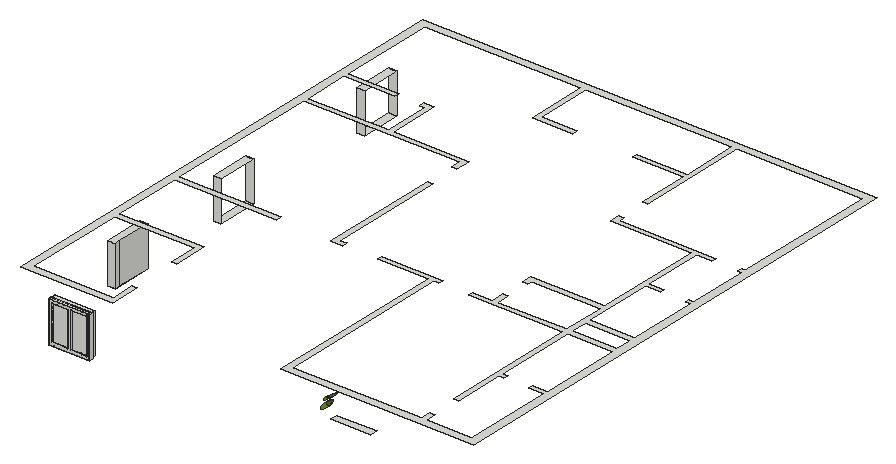
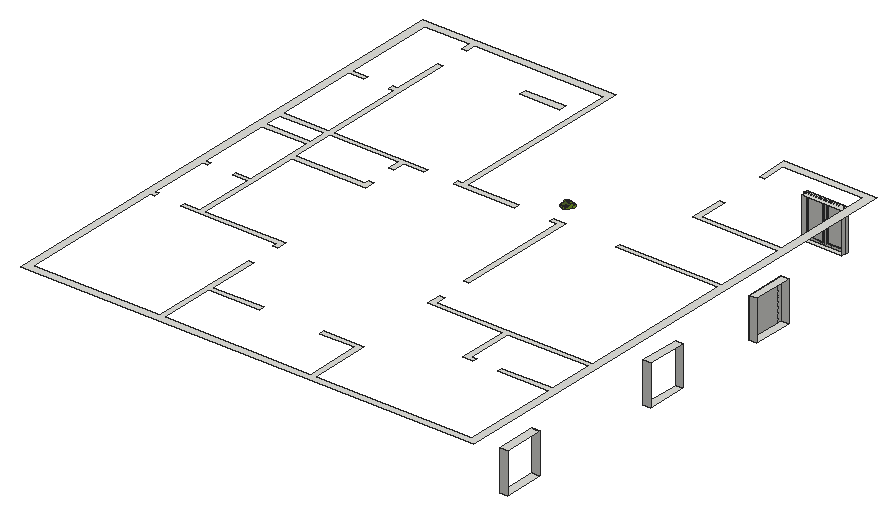
# SketchUp Ruby script. Lengths in inches.
U = 1.inch
M = Sketchup.active_model
def pt(a) = Geom::Point3d.new(a.map { |v| v * U })
def face(e, loops, mat)
  f = e.add_face(loops[0].map { |a| pt(a) })
  loops[1..].each { |l| e.add_face(l.map { |a| pt(a) }).erase! }
  f.material = f.back_material = mat if mat
  f
end
# faces: each face lists its corners as indices into pts; further lists are holes
def faces(e, pts, list, mat = nil) = list.each { |f| face(e, (f[0].is_a?(Array) ? f : [f]).map { |l| l.map { |i| pts[i] } }, mat) }
# xy, xz, yz: faces in a plane at the given z, y or x. An outline is a flat list of corners, or four numbers for a rectangle; further outlines are holes
def ring(l) = l.size == 4 ? [[l[0], l[1]], [l[2], l[1]], [l[2], l[3]], [l[0], l[3]]] : l.each_slice(2).to_a
def flat(e, list, mat, &to3) = list.each { |f| face(e, (f[0].is_a?(Array) ? f : [f]).map { |l| ring(l).map { |u, v| to3.(u, v) } }, mat) }
def xy(e, z, list, mat = nil) = flat(e, list, mat) { |x, y| [x, y, z] }
def xz(e, y, list, mat = nil) = flat(e, list, mat) { |x, z| [x, y, z] }
def yz(e, x, list, mat = nil) = flat(e, list, mat) { |y, z| [x, y, z] }
def lines(e, pts, list) = list.each { |a, b| e.add_line(pt(pts[a]), pt(pts[b])) }
# prism: a flat outline (further loops are holes) pulled along v
def prism(e, loops, v, mat = nil)
  f = face(e, loops, mat); d = Geom::Vector3d.new(v.map { |x| x * U })
  f.pushpull(f.normal.samedirection?(d) ? d.length : -d.length)
end
def box(e, o, s, mat = nil) = prism(e, [[o, [o[0] + s[0], o[1], o[2]], [o[0] + s[0], o[1] + s[1], o[2]], [o[0], o[1] + s[1], o[2]]]], [0, 0, s[2]], mat)
def at(x, y, z, deg = 0) = Geom::Transformation.translation(pt([x, y, z])) * Geom::Transformation.rotation(ORIGIN, Z_AXIS, deg.degrees)
def axes(o, x, y, z) = Geom::Transformation.new([*x, 0, *y, 0, *z, 0, *pt(o).to_a, 1])
def part(name) = M.definitions.add(name)
# library, detail: a bought-in or finely detailed component or shape, given as its bounding box
def library(name, o, s) = part(name).tap { |d| box(d.entities, o, s) }
def detail(e, o, s) = box(e.add_group.entities, o, s)
def put(e, d, t, mat = nil) = e.add_instance(d, t).tap { |i| i.material = mat if mat }
def group(e, t, mat = nil) = e.add_group.tap { |g| g.transformation = t; g.material = mat if mat }.entities
root = M.entities
M.materials.add("[0059_DarkOliveGreen]").color = [85, 107, 47]
M.materials.add("[0061_OliveDrab]").color = [107, 142, 35]
c1 = part("Window")
xy(c1.entities,31.72,[[-0.78,88.6,2.72,128.1]])
xy(c1.entities,34.95,[[-0.78,91.53,0.84,106.59],[0.84,91.53,1.05,97.58],[1.05,91.53,1.42,106.59],[1.42,91.53,2.72,106.59],[0.84,97.58,1.05,98.18],
  [0.84,98.18,1.05,106.59]])
xy(c1.entities,35.27,[[-0.78,110.09,0.97,125.14],[1.05,110.09,2.72,125.14]])
xy(c1.entities,58.35,[[2.72,108.74,3.8,109.74]])
xy(c1.entities,77.8125,[[-0.78,110.09,2.72,125.14],[0.97,110.09,1.05,125.14]])
xy(c1.entities,77.93,[[-0.78,91.53,0.84,106.59],[1.05,91.53,1.42,106.59],[1.42,91.53,2.72,106.59]])
xy(c1.entities,80.72,[[-0.78,88.6,2.72,128.1]])
xz(c1.entities,88.6,[[-0.78,31.72,2.72,80.72]])
xz(c1.entities,91.53,[[-0.78,34.95,0.84,77.93],[1.05,34.95,1.42,77.93],[1.42,34.95,2.72,77.93]])
xz(c1.entities,106.59,[[-0.78,34.95,0.84,77.93],[0.84,34.95,1.05,77.93],[0.84,34.95,2.72,77.93]])
xz(c1.entities,108.74,[[3.8,54.35,4.22,54.6,4.22,59.47,2.72,59.97,2.72,58.35,3.8,58.35]])
xz(c1.entities,109.74,[[3.8,54.35,3.8,58.35,2.72,58.35,2.72,59.97,4.22,59.47,4.22,54.6]])
xz(c1.entities,110.09,[[-0.78,35.27,0.97,77.8125],[1.05,35.27,2.72,77.8125]])
xz(c1.entities,125.14,[[-0.78,35.27,0.97,77.8125],[0.97,35.27,1.05,80.72],[1.05,35.27,2.72,77.8125]])
xz(c1.entities,128.1,[[-0.78,31.72,2.72,80.72]])
yz(c1.entities,-0.78,[[[88.6,31.72,128.1,80.72],[91.53,34.95,106.59,77.93],[110.09,35.27,125.14,77.8125]]])
yz(c1.entities,0.84,[[91.53,34.95,106.59,77.93]])
yz(c1.entities,0.97,[[110.09,35.27,125.14,77.8125]])
yz(c1.entities,1.05,[[91.53,34.95,106.59,77.93],[110.09,35.27,125.14,77.8125]])
yz(c1.entities,1.42,[[91.53,34.95,106.59,77.93]])
yz(c1.entities,2.72,[[[88.6,31.72,108.35,80.72],[91.53,34.95,106.59,77.93]],[[108.35,31.72,128.1,80.72],[110.09,35.27,125.14,77.8125],[108.74,58.35,109.74,59.97]]])
yz(c1.entities,3.8,[[108.74,54.35,109.74,58.35]])
yz(c1.entities,4.22,[[108.74,54.6,109.74,59.47]])
p = [[4.22,108.74,54.6],[3.8,108.74,54.35],[3.8,109.74,54.35],[4.22,109.74,54.6],[2.72,109.74,59.97],[2.72,108.74,59.97],
  [4.22,108.74,59.47],[4.22,109.74,59.47],[-0.78,86.4,89.94],[-0.78,86.44,89.94],[15.22,130.69,89.94],[15.22,130.65,89.94],
  [-0.78,86.44,28.19],[-0.78,86.4,28.19],[7.72,130.69,89.94],[7.72,130.65,89.94]]
faces(c1.entities,p,[[0,1,2,3],[4,5,6,7]])
lines(c1.entities,p,[[8,9],[10,11],[12,13],[14,15]])
xy(root,30.79,[[0,130.58,9,178.58],[0,288.02,9,336.02],[0,501.46,9,549.46]])
xy(root,38.11,[[33.63,0,81.63,9]])
xy(root,75.37,[[370.05,0,418.05,9]])
xy(root,78.79,[[0,130.58,9,178.58],[0,288.02,9,336.02],[0,501.46,9,549.46]])
xy(root,86.11,[[33.63,0,81.63,9]])
xy(root,108,[[[0,0,110,0,110,36.625,104,36.625,104,9,9,9,9,130,104,130,104,95.625,110,95.625,110,136,9,136,9,219,130,219,130,225,9,225,9,411,195,411,195,399,201,399,201,417,111,417,111,477,99,477,99,471,105,471,105,417,9,417,9,471,69,471,69,477,9,477,9,591,195,591,195,519,243.14,519,243.14,525,201,525,201,591,375,591,375,525,315.14,525,315.14,519,375,519,375,459,381,459,381,591,531,591,531,417,526.66,417,526.66,411,531,411,531,340,525,340,525,335,531,335,531,252,477,252,477,335,495,335,495,340,477,340,477,411,495.74,411,495.74,417,381,417,381,423,375,423,375,411,471,411,471,282,383,282,383,270,389,270,389,276,471,276,471,225,389,225,389,240,383,240,383,225,359,225,359,219,471,219,471,57,477,57,477,116,483,116,483,122,477,122,477,219,531,219,531,122,513,122,513,116,531,116,531,9,477,9,477,21,471,21,471,9,317,9,317,219,323,219,323,225,250.53,225,250.53,219,311,219,311,0,540,0,540,600,0,600],[477,225,531,246]],[195,219,208.87,219,208.87,225,201,225,201,363,195,363]])
xz(root,130.58,[[0,30.79,9,78.79]])
xz(root,178.58,[[0,30.79,9,78.79]])
xz(root,288.02,[[0,30.79,9,78.79]])
xz(root,336.02,[[0,30.79,9,78.79]])
xz(root,501.46,[[0,30.79,9,78.79]])
xz(root,549.46,[[0,30.79,9,78.79]])
yz(root,9,[[130.58,30.79,136,78.79],[136,30.79,178.58,78.79]])
yz(root,33.63,[[0,38.11,9,86.11]])
yz(root,81.63,[[0,38.11,9,86.11]])
p = [[303.91,81.51,31.81],[304.14,80.48,31.67],[304.01,79.54,31.42],[303.76,79.01,31.21],[303.29,78.55,30.94],[303.13,78.34,30.84],
  [303.1,79.46,31.08],[302.88,80.62,31.25],[302.55,81.73,31.37],[302.14,82.53,31.4],[302.01,82.68,31.38],[301.96,82.62,31.35],
  [302.02,82.34,31.3125],[302.4375,81.03,31.18],[302.71,79.875,31.03],[302.94,78.63,30.84],[303.01,77.97,30.72],[302.91,77.39,30.56],
  [302.67,77.08,30.41],[302.28,76.75,30.2],[301.93,76.47,30.01],[301.74,76.33,29.91],[301.4375,75.8125,29.69],[301.09,75.45,29.49],
  [300.73,75.23,29.31],[300.54,75.08,29.21],[300.5625,75.71,29.36],[300.6,76.66,29.57],[300.24,74.96,29.08],[300.13,74.76,29],
  [299.8,74.7,28.87],[299.47,74.65,28.73],[298.7,75.08,28.56],[297.62,75.29,28.21],[297.18,76.34,28.29],[296.74,77.08,28.29],
  [296.46,77.49,28.28],[297.01,78.56,28.7],[297.43,79.14,28.98],[298.05,79.55,29.29],[298.48,79.8,29.5],[298.6875,80.09,29.64],
  [298.86,80.33,29.75],[298.86,80.48,29.78],[298.74,80.54,29.75],[298.4,80.41,29.6],[298.12,80.21,29.46],[297.52,79.55,29.1],
  [297.02,78.96,28.8],[296.71,78.63,28.61],[296.5,78.25,28.46],[296.35,77.84,28.3125],[296.125,78.48,28.37],[296.02,79.02,28.45],
  [295.96,79.5,28.53],[295.9375,79.89,28.61],[295.88,80.34,28.6875],[296.37,81.17,29.04],[296.83,81.62,29.3],[297.24,81.82,29.49],
  [298,82.06,29.8125],[298.57,82.12,30.03],[299.0625,82.22,30.23],[299.42,82.36,30.39],[299.6,82.6,30.5],[299.61,82.92,30.58],
  [299.33,83.05,30.51],[298.96,83.14,30.39],[298.31,82.98,30.125],[297.6,82.57,29.78],[296.82,81.9375,29.37],[295.94,80.96,28.84],
  [295.84,82.59,29.16],[295.83,83.55,29.36],[295.97,83.97,29.5],[296.29,84.41,29.71],[296.68,84.67,29.91],[297.22,84.77,30.12],
  [297.67,84.84,30.3],[298.34,84.92,30.56],[298.83,84.87,30.72],[299.22,84.82,30.85],[299.41,84.76,30.9],[299.52,84.91,30.97],
  [299.4,85.13,30.98],[299.12,85.42,30.94],[298.67,85.56,30.8125],[297.76,85.4375,30.46],[297.22,85.26,30.23],[296.75,85.02,30.01],
  [296.53,84.79,29.88],[296.09,84.42,29.64],[296.07,84.68,29.7],[296.18,85.62,29.9375],[296.3,86.45,30.16],[296.74,87.4,30.52],
  [297.2,87.58,30.72],[297.94,87.44,30.96],[298.59,87.05,31.11],[299.19,86.76,31.26],[299.45,86.61,31.32],[299.6,86.64,31.38],
  [299.58,86.81,31.41],[299.28,87.16,31.38],[298.55,87.65,31.22],[297.96,87.8,31.04],[297.01,87.79,30.71],[297.49,88.92,31.12],
  [297.97,89.5,31.42],[298.37,89.6,31.58],[298.58,89.41,31.61],[299.21,88.79,31.7],[299.67,88.22,31.75],[300.03,87.86,31.8],
  [300.18,87.82,31.84],[300.22,87.97,31.89],[300.15,88.13,31.9],[299.5625,88.88,31.85],[299.09,89.3125,31.78],[298.68,89.59,31.6875],
  [298.36,89.78,31.62],[298.75,90.2,31.85],[299.11,90.32,32],[299.58,90.14,32.13],[300.02,89.78,32.21],[300.47,89.53,32.32],
  [300.7,89.07,32.3],[301.09,88.52,32.32],[301.42,87.875,32.3],[301.58,87.02,32.17],[301.53,86.13,31.96],[301.42,85.61,31.81],
  [301.65,85.42,31.85],[301.84,85.85,32.01],[302.16,86.29,32.22],[302.57,86.26,32.36],[303.18,85.93,32.5],[303.73,85.6,32.63],
  [304.125,85.47,32.74],[304.36,83.6,32.42],[304.35,82.48,32.17],[304.15,81.83,31.96],[302.35,78.69,30.64],[302.07,81.12,31.07],
  [301.58,82.73,31.24],[301.05,84.09,31.35],[301.19,84.49,31.48],[301.73,83.94,31.56],[302.45,83.22,31.66],[303.17,81.58,31.56],
  [302.67,83.06,31.7],[302.11,84.15,31.74],[301.47,84.58,31.6],[301.37,84.78,31.61],[301.58,85.07,31.75],[302.58,84.5,31.98],
  [303.72,84.24,32.33],[301.46,85.37,31.77],[301.27,86.02,31.84],[300.98,87.4375,32.04],[300.59,88.32,32.1],[300.25,88.84,32.09],
  [300.78,87.35,31.95],[301.08,86.13,31.8],[301.18,85.44,31.68],[300.75,86.54,31.77],[299.91,87.57,31.6875],[299.23,88.12,31.57],
  [298.53,88.54,31.41],[298.19,88.67,31.3125],[299.26,87.8125,31.51],[299.9,87.21,31.61],[300.61,86.39,31.68],[300.97,85.68,31.66],
  [301.12,85.28,31.63],[301.09,85.03,31.5625],[300.97,84.97,31.51],[300.66,85.21,31.45],[300.34,85.6,31.42],[299.97,85.85,31.34],
  [298.9,86.35,31.07],[298.22,86.5,30.86],[297.58,86.36,30.6],[297.06,86.27,30.39],[296.86,86,30.26],[297.86,86.19,30.66],
  [298.43,86.13,30.85],[299.33,85.85,31.11],[300.12,85.39,31.29],[300.98,84.75,31.46],[300.53,83.74,31.08],[299.86,83.98,30.9],
  [299.23,84.18,30.72],[297.93,83.99,30.21],[297.28,83.64,29.9],[296.85,83.33,29.68],[296.65,83.05,29.55],[297.26,83.38,29.84],
  [298.27,83.68,30.26],[299.56,83.77,30.74],[300.33,83.47,30.95],[299.64,81.54,30.29],[299.12,81.68,30.13],[298.48,81.48,29.86],
  [297.875,81.06,29.55],[297.41,80.6,29.29],[296.91,79.91,28.96],[297.95,80.89,29.54],[298.56,81.28,29.85],[299.12,81.41,30.08],
  [299.63,81.3125,30.24],[299.19,79.81,29.75],[298.63,79.54,29.5],[298.13,79.07,29.22],[297.72,78.51,28.95],[297.54,77.96,28.76],
  [298.23,78.9,29.21],[298.74,79.27,29.48],[299.16,79.49,29.67],[298.73,78.33,29.27],[298.51,77.7,29.05],[298.1875,76.91,28.77],
  [298.25,77.01,28.81],[298.86,78.18,29.28],[299.35,79.38,29.72],[299.73,80.8,30.16],[299.98,77.43,29.52],[299.97,81.28,30.35],
  [300.41,82.42,30.76],[300.8125,80.77,30.54],[301.22,78.1,30.11],[301.07,80.07,30.48],[300.77,81.88,30.77],[300.53,82.84,30.89],
  [300.96,83.8,31.25],[301.66,81.72,31.05],[301.66,80.23,30.73],[301.42,81.35,30.88],[301.3,81.62,30.9],[301.21,81.68,30.88],
  [301.17,81.56,30.84],[301.24,81.11,30.77],[301.42,80.05,30.6],[301.61,78.875,30.41],[301.75,77.64,30.2],[301.83,77.06,30.1],
  [301.8,78.81,30.47],[300.55,80.37,30.36],[300.4375,80.76,30.41],[300.31,80.79,30.36],[300.24,80.61,30.3],[300.23,80.22,30.21],
  [300.27,79.91,30.16],[300.4375,78.67,29.95],[300.6,77.52,29.76],[300.62,79.28,30.15],[303.56,82.63,31.93],[303.37,83.17,31.97],
  [303.05,83.66,31.96],[302.77,83.9375,31.93],[302.62,83.91,31.87],[302.57,83.78,31.82],[303.04,82.94,31.81],[303.45,82.28,31.8125],
  [303.57,82.16,31.83],[300.01,84.53,31.07],[300.24,84.3,31.1],[300.52,84.35,31.21],[300.61,84.6,31.3],[300.42,84.84,31.28],
  [300.18,84.89,31.21],[300,84.74,31.11],[300.84,85.67,31.61],[300.59,85.84,31.56],[300.4,85.85,31.49],[300.41,85.64,31.45],
  [300.68,85.45,31.51],[300.88,85.4375,31.57],[300.28,89.38,36.32],[300.2,89.78,36.28],[300.5,90.01,36.43],[300.92,90.59,36.64],
  [301.17,91.375,36.77],[301.21,92.22,36.79],[301.18,93.06,36.77],[301.21,93.65,36.79],[301,94.35,36.68],[300.84,95.125,36.6],
  [300.58,95.8,36.47],[300.27,96.13,36.32],[299.82,96.3,36.09],[299.96,95.79,36.16],[300.14,95.11,36.25],[300.29,94.26,36.32],
  [300.375,93.04,36.37],[300.36,92.84,36.36],[300.27,92.78,36.3125],[300.18,92.98,36.27],[300.08,93.66,36.22],[299.99,94.61,36.18],
  [299.82,95.78,36.09],[299.75,96.15,36.05],[299.43,96.55,35.89],[298.83,96.7,35.59],[298.02,96.46,35.18],[298.6875,95.36,35.52],
  [299.04,94.57,35.7],[299.35,93.37,35.85],[299.41,92.77,35.88],[299.35,92.63,35.85],[299.23,92.78,35.79],[299.11,93.19,35.73],
  [298.82,94.09,35.58],[298.52,95.13,35.43],[298.06,96.09,35.2],[297.65,96.5,34.99],[296.93,96.35,34.63],[296.5,95.89,34.41],
  [296.02,95.36,34.17],[295.92,95.15,34.12],[296.06,94.91,34.1875],[296.39,94.9,34.35],[296.64,94.81,34.48],[297.08,94.42,34.7],
  [297.53,93.93,34.93],[298.23,92.95,35.28],[298.49,92.33,35.41],[298.57,91.79,35.45],[298.55,91.5,35.45],[298.41,91.52,35.375],
  [298.3,91.78,35.32],[298.05,92.27,35.19],[297.72,92.88,35.03],[297.21,93.61,34.77],[296.86,94.08,34.59],[296.44,94.63,34.38],
  [295.64,94.98,33.98],[295.36,94.84,33.83],[294.96,94.15,33.63],[294.33,92.88,33.3125],[295.37,92.54,33.84],[296.19,92.08,34.26],
  [296.87,91.55,34.59],[297.4,90.89,34.86],[297.625,90.4,34.98],[297.76,89.98,35.05],[297.62,89.77,34.97],[297.39,89.8,34.86],
  [297.08,90.13,34.7],[296.6875,90.63,34.51],[296.25,91.26,34.28],[295.62,91.97,33.96],[295.24,92.3,33.77],[294.72,92.53,33.51],
  [294.02,92.51,33.16],[293.87,92.12,33.08],[293.72,91.82,33.01],[293.55,91.41,32.92],[293.39,90.91,32.84],[293.28,90.2,32.78],
  [293.5625,90.31,32.93],[293.875,90.34,33.08],[294.24,90.2,33.27],[294.84,90.04,33.57],[295.54,89.81,33.93],[295.84,89.62,34.08],
  [296.13,89.31,34.22],[296.1875,89.14,34.25],[296.12,89.03,34.22],[295.9,89.06,34.11],[295.63,89.1,33.97],[295.21,89.43,33.76],
  [294.61,89.85,33.45],[294.06,89.9375,33.17],[293.21,89.82,32.75],[293.23,89.2,32.76],[293.23,88.17,32.76],[293.09,86.91,32.6875],
  [293.76,85.5,33.03],[294.12,84.3,33.21],[294.38,83.95,33.34],[294.64,83.61,33.47],[294.8,83.63,33.55],[295.78,84.41,34.05],
  [295.35,83.77,33.83],[295.06,83.36,33.68],[295.26,83.24,33.78],[295.6,82.98,33.96],[296.01,82.83,34.16],[296.45,82.83,34.38],
  [296.64,82.72,34.48],[297.01,82.5,34.67],[297.43,82.29,34.88],[297.73,82.23,35.03],[298.04,82.52,35.1875],[298.28,83.07,35.31],
  [298.65,84.21,35.5],[298.95,85.35,35.65],[299.22,86.77,35.78],[299.3,87.03,35.82],[299.36,87.02,35.85],[299.38,86.76,35.87],
  [299.33,85.71,35.84],[299.09,84.54,35.72],[298.75,83.47,35.55],[298.29,82.64,35.3125],[298.49,82.61,35.42],[299.02,82.39,35.68],
  [299.43,82.47,35.89],[299.93,82.97,36.14],[300.2,83.97,36.28],[300.5,83.92,36.43],[300.92,84.15,36.64],[301.41,84.92,36.89],
  [302.05,86.52,37.21],[301.83,87.08,37.1],[301.58,87.95,36.97],[301.29,88.89,36.83],[301.01,89.4,36.6875],[300.59,89.46,36.48],
  [297.32,88.4,34.82],[295.67,85.68,33.99],[296.9375,88.36,34.63],[296.0625,87.78,34.19],[295.2,87.51,33.76],[294.27,87.4,33.28],
  [294.18,87.39,33.24],[294.75,87.58,33.52],[295.17,87.76,33.74],[295.97,88.09,34.14],[295.59,88.42,33.95],[295.0625,88.76,33.68],
  [294.18,88.89,33.24],[294.54,89.07,33.42],[295.07,88.99,33.6875],[295.62,88.73,33.97],[296.13,88.27,34.23],[297.09,88.82,34.71],
  [296.77,89.49,34.55],[296.32,90.05,34.32],[295.72,90.48,34.02],[294.5625,91.01,33.43],[295.22,90.91,33.76],[295.74,90.69,34.02],
  [296.35,90.28,34.33],[296.88,89.68,34.6],[297.19,88.98,34.76],[298.51,89.53,35.42],[298.09,90.65,35.21],[297.14,92.09,34.73],
  [296.3,93.06,34.31],[295.73,93.53,34.02],[295.99,93.49,34.15],[296.43,93.21,34.37],[297.03,92.71,34.68],[298.04,91.32,35.1875],
  [298.4,90.44,35.37],[298.77,89.49,35.56],[299.52,89.68,35.93],[299.18,91.14,35.76],[298.82,92.39,35.58],[298.31,93.63,35.32],
  [297.93,94.33,35.13],[297.14,95.37,34.73],[297.39,95.33,34.86],[297.8,94.79,35.07],[298.32,94.14,35.33],[298.73,93.23,35.54],
  [299.28,91.64,35.8125],[299.43,91.02,35.89],[299.49,90.39,35.92],[299.61,89.85,35.98],[299.71,89.76,36.03],[299.84,89.89,36.1],
  [299.91,90.35,36.13],[299.96,91.28,36.16],[299.81,92.68,36.08],[299.62,93.85,35.98],[299.22,95.71,35.78],[299.41,95.21,35.88],
  [299.72,94.1,36.04],[299.97,92.93,36.16],[300.12,91.21,36.24],[299.95,89.9375,36.15],[300.18,90.54,36.27],[300.49,91.76,36.43],
  [300.76,93.42,36.56],[300.77,92.66,36.57],[300.67,91.58,36.52],[300.27,90.24,36.32],[300.12,89.55,36.24],[301.24,86.12,36.8],
  [300.54,87.63,36.45],[300.08,89.21,36.22],[299.81,89.25,36.08],[299.79,88.99,36.07],[300.0625,87.94,36.21],[299.99,86.51,36.17],
  [299.71,84.89,36.03],[299.9,86.89,36.13],[299.7,88.24,36.03],[299.56,89.25,35.95],[299.28,89.14,35.82],[299.08,87.55,35.71],
  [298.73,85.84,35.54],[297.89,83.8,35.11],[298.7,86.74,35.52],[299.1,89.03,35.72],[298.38,88.86,35.36],[298.14,87.9,35.24],
  [297.58,86.26,34.95],[296.83,84.7,34.58],[297.69,87.0625,35.01],[298.12,88.7,35.23],[298.0625,85.69,35.2],[297.74,84.94,35.03],
  [297.56,84.52,34.94],[296.82,83.26,34.57],[297.01,83.75,34.67],[297.44,84.8,34.89],[297.8125,85.84,35.07],[298.14,86.8,35.24],
  [298.28,87.2,35.3125],[298.36,87.24,35.35],[298.4,87.1,35.37],[298.37,86.76,35.36],[297.13,86.66,34.73],[297.02,86.44,34.67],
  [296.92,86.23,34.62],[296.15,85.02,34.23],[296.53,86.01,34.42],[296.94,87.09,34.63],[297.04,87.36,34.68],[297.22,87.625,34.77],
  [297.34,87.66,34.84],[297.42,87.5,34.875],[297.33,87.08,34.83],[300.52,86.14,36.44],[300.53,85.78,36.44],[300.4375,85.17,36.4],
  [300.24,84.82,36.3],[300.21,85.05,36.28],[300.2,86,36.28],[300.23,87.14,36.29],[300.31,87.18,36.34],[300.43,87.02,36.4],
  [300.51,86.5,36.4375],[299.02,89.93,35.68],[298.8,90.23,35.57],[298.74,90.65,35.54],[298.82,90.82,35.58],[299.01,90.71,35.68],
  [299.16,90.4,35.75],[299.19,90.01,35.77],[299.74,90.79,36.05],[299.8125,90.5,36.08],[299.74,90.29,36.05],[299.61,90.53,35.98],
  [299.49,90.97,35.92],[299.58,91.13,35.97],[299.71,90.91,36.03],[299.01,90.72,35.68]]
faces(root,p,[[[0,1,2,3,4,5,6,7,8,9,10,11,12,13,14,15,16,17,18,19,20,21,22,23,24,25,26,27,28,29,30,31,32,33,34,35,36,37,38,39,40,41,42,43,44,45,46,47,48,49,50,51,52,53,54,55,56,57,58,59,60,61,62,63,64,65,66,67,68,69,70,71,72,73,74,75,76,77,78,79,80,81,82,83,84,85,86,87,88,89,90,75,91,92,93,94,95,96,97,98,99,100,101,102,103,104,105,106,107,108,109,110,111,112,113,114,115,116,117,118,119,120,121,122,123,124,125,126,127,128,129,130,131,132,133,134,135,136,137,138,139,140,141],[142,143,144,145,146,147,148,149,150,151,152,153,154,155,156,157,158,159,160,161,162,163,164,165,166,167,168,169,170,171,172,173,174,175,176,177,178,179,180,181,182,183,184,185,186,187,188,189,190,191,192,193,194,195,196,197,198,199,200,201,202,203,204,205,206,207,208,209,210,211,212,213,214,215,216,217,218,219,220,221,222,223,224,225,226,227,228,229,230,231,232,233,234,235],[236,237,238,239,240,241,242,243,244,245,246],[247,248,249,250,251,252,253,254,255],[256,257,258,259,260,261,262,263,264],[265,266,267,268,269,270,271],[272,273,274,275,276,277]],[[278,279,280,281,282,283,284,285,286,287,288,289,290,291,292,293,294,295,296,297,298,299,300,301,302,303,304,305,306,307,308,309,310,311,312,313,314,315,316,317,318,319,320,321,322,323,324,325,326,327,328,329,330,331,332,333,334,335,320,336,337,338,339,340,341,342,343,344,345,346,347,348,349,350,351,352,353,354,355,356,357,358,359,360,361,362,363,364,365,366,367,368,369,370,371,372,373,374,375,376,377,378,379,380,381,382,383,384,385,386,387,388,389,390,391,392,393,394,395,396,397,398,399,400,401,402,403,404,405,406,407,408,409,410,411,412,413,414,415,416,417,418,419],[420,421,422,423,424,425,426,427,428,429,430,431,432,433,434,435,436,437,438,439,440,441,442,443,444,445,446,447,448,449,450,451,452,453,454,455,456,457,458,459,460,461,462,463,464,465,466,467,468,469,470,471,472,473,474,475,476,477,478,479,480,481,482,483,484,485,486,487,488,489,490,491,492,493,494,495,496,497,498,499,500,501,502,503,504,505,506,507,508,509,510,511,512,513],[514,515,516,517,518,519,520,521,522,523,524,525],[526,527,528,529,530,531,532,533,534,535,536],[537,538,539,540,541,542,543,544,545,546],[547,548,549,550,551,552,553],[554,555,556,557,558,559,560]]],"[0061_OliveDrab]")
faces(root,p,[[143,142,235,234,233,232,231,230,229,228,227,226,225,224,223,222,221,220,219,218,217,216,215,214,213,212,211,210,209,208,207,206,205,204,203,202,201,200,199,198,197,196,195,194,193,192,191,190,189,188,187,186,185,184,183,182,181,180,179,178,177,176,175,174,173,172,171,170,169,168,167,166,165,164,163,162,161,160,159,158,157,156,155,154,153,152,151,150,149,148,147,146,145,144],[421,420,513,512,511,510,509,508,507,506,505,504,503,502,501,500,499,498,497,496,495,494,493,492,491,490,489,488,487,486,485,484,483,482,481,480,479,478,477,476,475,474,473,472,471,470,469,468,467,466,465,464,463,462,461,460,459,458,457,456,455,454,453,452,451,450,449,448,447,446,445,444,443,442,441,440,439,438,437,436,435,434,433,432,431,430,429,428,427,426,425,424,423,422]],"[0059_DarkOliveGreen]")
lines(root,p,[[551,561]])
put(root,c1,axes([193.75,0.78,5.38],[0,1,0],[-1.25,0,0],[0,0,1]))
